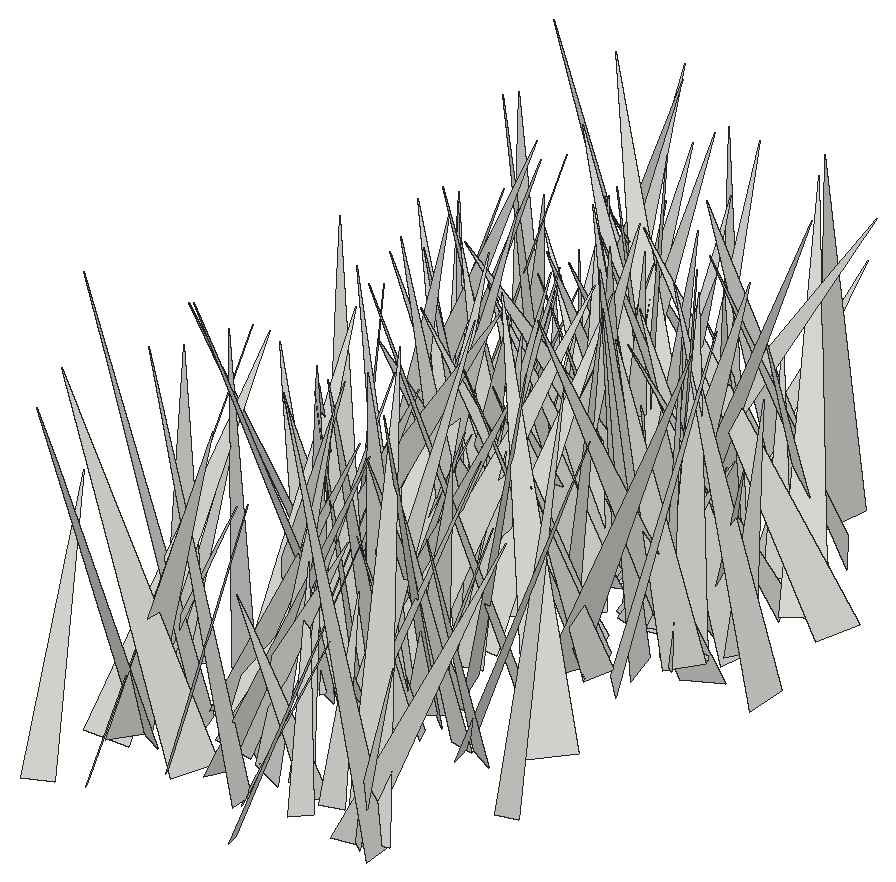
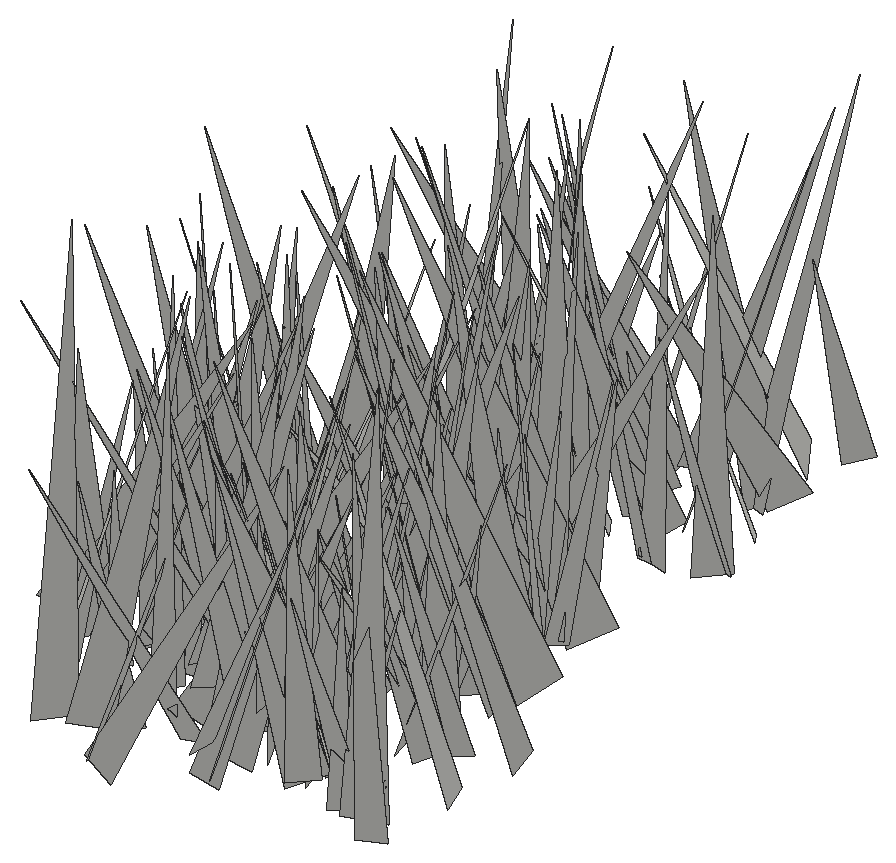
# SketchUp Ruby script. Lengths in inches.
U = 1.inch
M = Sketchup.active_model
def pt(a) = Geom::Point3d.new(a.map { |v| v * U })
def face(e, loops, mat)
  f = e.add_face(loops[0].map { |a| pt(a) })
  loops[1..].each { |l| e.add_face(l.map { |a| pt(a) }).erase! }
  f.material = f.back_material = mat if mat
  f
end
# faces: each face lists its corners as indices into pts; further lists are holes
def faces(e, pts, list, mat = nil) = list.each { |f| face(e, (f[0].is_a?(Array) ? f : [f]).map { |l| l.map { |i| pts[i] } }, mat) }
# xy, xz, yz: faces in a plane at the given z, y or x. An outline is a flat list of corners, or four numbers for a rectangle; further outlines are holes
def ring(l) = l.size == 4 ? [[l[0], l[1]], [l[2], l[1]], [l[2], l[3]], [l[0], l[3]]] : l.each_slice(2).to_a
def flat(e, list, mat, &to3) = list.each { |f| face(e, (f[0].is_a?(Array) ? f : [f]).map { |l| ring(l).map { |u, v| to3.(u, v) } }, mat) }
def xy(e, z, list, mat = nil) = flat(e, list, mat) { |x, y| [x, y, z] }
def xz(e, y, list, mat = nil) = flat(e, list, mat) { |x, z| [x, y, z] }
def yz(e, x, list, mat = nil) = flat(e, list, mat) { |y, z| [x, y, z] }
def lines(e, pts, list) = list.each { |a, b| e.add_line(pt(pts[a]), pt(pts[b])) }
# prism: a flat outline (further loops are holes) pulled along v
def prism(e, loops, v, mat = nil)
  f = face(e, loops, mat); d = Geom::Vector3d.new(v.map { |x| x * U })
  f.pushpull(f.normal.samedirection?(d) ? d.length : -d.length)
end
def box(e, o, s, mat = nil) = prism(e, [[o, [o[0] + s[0], o[1], o[2]], [o[0] + s[0], o[1] + s[1], o[2]], [o[0], o[1] + s[1], o[2]]]], [0, 0, s[2]], mat)
def at(x, y, z, deg = 0) = Geom::Transformation.translation(pt([x, y, z])) * Geom::Transformation.rotation(ORIGIN, Z_AXIS, deg.degrees)
def axes(o, x, y, z) = Geom::Transformation.new([*x, 0, *y, 0, *z, 0, *pt(o).to_a, 1])
def part(name) = M.definitions.add(name)
# library, detail: a bought-in or finely detailed component or shape, given as its bounding box
def library(name, o, s) = part(name).tap { |d| box(d.entities, o, s) }
def detail(e, o, s) = box(e.add_group.entities, o, s)
def put(e, d, t, mat = nil) = e.add_instance(d, t).tap { |i| i.material = mat if mat }
def group(e, t, mat = nil) = e.add_group.tap { |g| g.transformation = t; g.material = mat if mat }.entities
root = M.entities
c1 = part("fur_instance\#9")
p = [[0.8125,0,1.79],[0.67,-0.02,1.48],[0,-0.11,0],[0,0.11,0]]
faces(c1.entities,p,[[0,1,2,3]])
put(root,c1,axes([74.57,65.62,-28.22],[6.72772,1.76518,0.89994],[1.69777,-6.77807,0.60273],[-1.02144,0.36032,6.92927]))
put(root,c1,axes([76.2,71.65,-28.22],[2.05152,-6.96349,2.48946],[-7.36809,-2.14532,0.07104],[-0.63146,2.40909,7.25905]))
put(root,c1,axes([76.23,53.86,-27.1],[4.61817,-3.87726,2.02523],[-4.05143,-4.90172,-0.14567],[-1.64942,1.18414,6.02822]))
put(root,c1,axes([75.16,72.59,-28.22],[0.26156,-6.27199,1.2943],[-6.21893,0.06053,1.55008],[1.52905,1.31908,6.08306]))
put(root,c1,axes([77.24,45.125,-27.1],[-3.56448,3.67904,0.44666],[3.56023,3.5714,-1.00507],[1.02934,0.38746,5.02301]))
put(root,c1,axes([78.23,67.21,-28.22],[-5.39834,-1.72938,0.70035],[-1.70183,5.44274,0.32197],[0.76486,-0.09564,5.65943]))
put(root,c1,axes([79.26,51.24,-27.1],[-7.24522,-3.15461,1.03201],[-3.28219,7.17812,-1.10079],[0.49381,1.42581,7.82516]))
put(root,c1,axes([77.72,70.49,-28.22],[-2.1087,-2.96786,0.97974],[-3.12443,1.97245,-0.74971],[-0.07759,1.23123,3.56269]))
put(root,c1,axes([77.92,64.53,-27.1],[-4.02809,-0.22088,0.67447],[-0.39433,3.92835,-1.06856],[0.59008,1.11738,3.89005]))
put(root,c1,axes([76.2,53.45,-27.1],[1.29664,4.3065,0.97913],[4.41517,-1.23995,-0.39328],[0.1042,-1.05001,4.48024]))
put(root,c1,axes([74.85,68.74,-28.22],[6.72571,2.73267,0.89443],[2.78268,-6.75899,-0.27437],[-0.72399,-0.59256,7.25447]))
put(root,c1,axes([77.43,70.7,-28.22],[-0.62554,4.99616,0.12365],[4.99768,0.62512,0.02455],[-0.009,-0.12574,5.03511]))
put(root,c1,axes([78.375,57.875,-27.1],[-1.43576,4.62376,1.24523],[4.74317,1.1948,1.0324],[-0.65727,-1.47798,4.73019]))
put(root,c1,axes([77.3,60.48,-27.1],[-3.93498,0.71077,2.15609],[1.47172,4.08376,1.33974],[1.72857,-1.85895,3.76754]))
put(root,c1,axes([76.38,62.34,-27.1],[-4.16703,-2.76107,2.92288],[-2.78486,5.0182,0.77013],[2.90022,0.85149,4.93909]))
put(root,c1,axes([77.23,71.6,-28.22],[2.21811,-2.97156,1.30139],[-3.14682,-2.35396,-0.01147],[-0.78819,1.03561,3.7081]))
put(root,c1,axes([77.92,65.62,-28.22],[-2.20554,5.93145,2.00046],[6.2413,2.24627,0.22087],[0.47966,-1.95462,6.32437]))
put(root,c1,axes([75.81,71.11,-27.1],[3.73133,2.74864,1.27928],[3.02044,-3.19509,-1.94493],[0.26177,-2.31318,4.20655]))
put(root,c1,axes([76.375,66.4375,-28.22],[-0.11814,4.24138,1.60816],[4.31681,0.59918,-1.26317],[1.39308,-1.49704,4.05064]))
put(root,c1,axes([77.28,48.58,-27.1],[-4.67484,5.38464,0.57126],[4.73589,4.43174,-3.01759],[2.62527,1.59378,6.46085]))
put(root,c1,axes([76.33,64.45,-27.1],[6.99612,0.8962,1.32294],[0.53893,-6.91662,1.83548],[-1.5043,1.69005,6.81028]))
put(root,c1,axes([78.14,49.53,-27.1],[-2.86218,-6.85746,0.77217],[-6.83354,2.93291,0.71683],[0.96112,0.43167,7.39614]))
put(root,c1,axes([78.7,65.04,-27.1],[2.01081,5.29668,2.07869],[5.40677,-2.46554,1.0522],[-1.77275,-1.51176,5.56697]))
put(root,c1,axes([80.99,57.3,-27.1],[-3.56669,-5.90918,0.59479],[-5.71236,3.22345,-2.22975],[-1.62517,1.63841,6.53207]))
put(root,c1,axes([79.25,68.78,-27.1],[-6.68963,-2.36331,2.10659],[-2.62997,6.88987,-0.62215],[1.76244,1.31094,7.06748]))
put(root,c1,axes([77.18,67.32,-28.22],[3.08965,-1.86478,1.07968],[-2.12915,-2.93231,1.02827],[-0.33144,1.45368,3.45919]))
put(root,c1,axes([75.82,63.17,-27.1],[7.81962,-2.04899,1.63917],[-2.46618,-7.49875,2.3913],[-0.8962,2.75717,7.72182]))
put(root,c1,axes([78.22,54.46,-27.1],[-1.72933,-6.01967,2.37326],[-6.41752,1.90965,0.16749],[0.82719,2.23073,6.26091]))
put(root,c1,axes([77.84,66.42,-27.1],[3.89032,1.8987,0.46131],[1.51623,-3.58179,1.95558],[-1.23244,1.58688,3.86204]))
put(root,c1,axes([80.93,73.32,-27.1],[-7.3033,-3.33888,1.09507],[-3.45877,7.27632,-0.88176],[0.61989,1.26191,7.98178]))
put(root,c1,axes([76.66,51.13,-27.1],[3.8277,2.64651,0.3376],[2.6435,-3.68235,-1.10521],[0.36045,-1.09797,4.52038]))
put(root,c1,axes([78.35,60.38,-27.1],[0.55845,-3.67703,0.59896],[-3.72525,-0.55803,0.04757],[-0.0423,0.59936,3.71889]))
put(root,c1,axes([80.03,63.82,-27.1],[-2.9661,5.6248,1.68099],[5.86235,2.73802,1.18234],[-0.31135,-2.03143,6.24805]))
put(root,c1,axes([78.06,72.44,-27.1],[3.7544,-3.60472,1.46029],[-3.77286,-3.86843,0.15082],[-0.94444,1.12393,5.20257]))
put(root,c1,axes([80.8,48.69,-27.1],[-5.74656,4.30747,2.03787],[4.75581,5.38477,2.02895],[0.29923,-2.86007,6.88916]))
put(root,c1,axes([79.17,70.58,-28.22],[-4.422,-0.95671,1.75223],[-1.16644,4.69405,-0.38074],[1.6202,0.76828,4.50826]))
put(root,c1,axes([77.58,62.09,-27.1],[6.54433,-2.87567,1.841],[-3.10892,-6.66403,0.64215],[-1.41189,1.3447,7.11937]))
put(root,c1,axes([77.62,62.73,-27.1],[3.69637,0.13401,0.11411],[0.12786,-3.69317,0.19555],[-0.12096,0.19138,3.69362]))
put(root,c1,axes([77.38,64.68,-27.1],[2.01974,-4.62687,0.27657],[-4.52399,-1.90214,1.21619],[1.00891,0.73329,4.89981]))
put(root,c1,axes([79.6,67.66,-28.22],[-6.44031,-4.10602,1.97316],[-3.85542,6.73281,1.42663],[2.42663,-0.20036,7.50344]))
put(root,c1,axes([79.36,65.3125,-27.1],[-5.69321,-2.11736,2.09192],[-1.78965,6.04293,1.24584],[2.37833,-0.52131,5.94506]))
put(root,c1,axes([80.4,67.98,-28.22],[-5.18821,0.426,1.12668],[0.56814,5.25845,0.62796],[1.06213,-0.73187,5.16766]))
put(root,c1,axes([77.65,60.375,-27.1],[-1.30326,-6.4856,0.41929],[-6.05179,1.36694,2.33336],[2.36951,-0.07596,6.19006]))
put(root,c1,axes([80.39,58.46,-27.1],[-1.23415,4.06964,0.18802],[4.01431,1.18128,0.78126],[-0.69473,-0.40381,4.18028]))
put(root,c1,axes([79.7,69.08,-28.22],[-7.05102,3.6652,1.50452],[2.87345,6.84526,-3.20935],[2.72774,2.26338,7.26985]))
put(root,c1,axes([78.58,46.01,-27.1],[6.47169,4.71895,0.84374],[4.29058,-6.33416,2.51645],[-2.13805,1.57262,7.60387]))
put(root,c1,axes([77.86,69.9,-27.1],[7.57177,-0.43303,1.80554],[-0.88332,-7.50835,1.90355],[-1.63317,2.05334,7.34137]))
put(root,c1,axes([82.125,57.54,-27.1],[-6.70082,0.16595,0.10129],[0.12128,6.29761,-2.29436],[0.15195,2.29157,6.29797]))
put(root,c1,axes([78.89,59.1,-27.1],[-1.68385,4.77561,0.18208],[4.53538,1.65768,-1.53538],[1.50664,0.34725,4.82539]))
put(root,c1,axes([80.23,59.44,-27.1],[-3.57041,1.71359,0.7726],[1.61509,3.64514,-0.62093],[0.96166,0.24019,3.91135]))
put(root,c1,axes([78.79,69.76,-28.22],[4.20297,-1.11156,0.80651],[-1.18233,-4.24977,0.30429],[-0.69867,0.5049,4.33681]))
put(root,c1,axes([81.92,72.79,-27.1],[-5.15429,0.32159,0.0951],[0.32057,5.15491,-0.05731],[0.09848,0.05128,5.164]))
put(root,c1,axes([77.75,49.14,-27.1],[6.355,-3.28716,0.66061],[-3.33311,-6.3472,0.48096],[-0.36352,0.73183,7.13864]))
put(root,c1,axes([77.41,58.91,-27.1],[3.81653,-4.78014,0.36891],[-4.62204,-3.54318,1.90641],[1.2738,1.46558,5.81217]))
put(root,c1,axes([81.25,55.76,-27.1],[-7.16118,3.19135,1.99245],[3.1192,7.43157,-0.69239],[2.1036,-0.15533,7.80947]))
put(root,c1,axes([81.09,70.15,-27.1],[-3.67286,3.55796,0.5072],[3.52102,3.70767,-0.51167],[0.72023,0.01818,5.08794]))
put(root,c1,axes([80.46,65.18,-27.1],[3.62515,-5.36286,0.15908],[-5.03579,-3.46731,-2.13211],[-1.85105,-1.06996,6.11196]))
put(root,c1,axes([79.2,70.78,-28.22],[5.50822,-3.47682,2.75588],[-4.25576,-5.38219,1.71589],[-1.25366,2.99458,6.28367]))
put(root,c1,axes([82.82,68.71,-28.22],[-3.6214,4.75768,0.36392],[4.63089,3.39426,1.70771],[-1.15013,-1.31374,5.73008]))
put(root,c1,axes([78.59,70.18,-28.22],[4.42426,3.38365,0.88099],[3.49585,-4.30744,-1.01209],[-0.06566,-1.34021,5.47712]))
put(root,c1,axes([80.74,65.16,-28.22],[-4.41847,1.33903,1.10997],[0.76139,4.21375,-2.05244],[1.56375,1.73183,4.13562]))
put(root,c1,axes([78.8125,60.33,-27.1],[3.29309,2.39527,0.08068],[2.3726,-3.23886,-0.68467],[0.3385,-0.60058,4.0141]))
put(root,c1,axes([81.21,64.29,-27.1],[3.41803,-2.18502,2.15563],[-1.95303,-4.03718,-0.99543],[-2.36786,0.1758,3.93273]))
put(root,c1,axes([80.29,52.21,-27.1],[-2.04424,6.85145,0.72305],[6.79433,2.1298,-0.97223],[1.1412,-0.40704,7.08351]))
put(root,c1,axes([83.23,48.0625,-27.1],[-7.26619,-2.16018,0.91047],[-2.32448,7.02333,-1.88745],[0.30351,2.07347,7.34176]))
put(root,c1,axes([81.4,61.94,-27.1],[-6.84332,-0.22544,2.15666],[-0.013,7.14388,0.70553],[2.16837,-0.66867,6.81058]))
put(root,c1,axes([81.04,58.81,-27.1],[-5.5806,3.5391,0.90465],[3.04631,5.42049,-2.4135],[2.01583,1.60617,6.15169]))
put(root,c1,axes([81.13,70.24,-28.22],[2.90611,1.79436,1.69144],[1.585,-3.36196,0.84331],[-1.88904,-0.06039,3.30969]))
put(root,c1,axes([79.44,60.96,-27.1],[7.05742,-1.09775,2.22467],[-1.64487,-7.09246,1.71837],[-1.85705,2.1103,6.93249]))
put(root,c1,axes([79.86,64.58,-28.22],[1.46502,-3.697,0.60293],[-3.73698,-1.39797,0.50827],[0.25762,0.74531,3.94408]))
put(root,c1,axes([78.72,64.59,-27.1],[3.57739,2.98141,0.96801],[3.07785,-3.06266,-1.94177],[0.59384,-2.08684,4.23274]))
put(root,c1,axes([76.67,59.43,-27.1],[6.17977,-5.38552,0.13557],[-5.06059,-5.73249,2.95646],[1.84733,2.31224,7.64543]))
put(root,c1,axes([81.78,71.32,-28.22],[0.31088,-6.10314,0.84199],[-6.04835,-0.46277,-1.12122],[-1.17245,0.76905,6.00731]))
put(root,c1,axes([82.6,63.05,-27.1],[-2.33709,5.71521,1.48586],[5.84354,2.00796,1.46781],[-0.85111,-1.90732,5.99759]))
put(root,c1,axes([81.27,70,-27.1],[-2.39364,-3.13142,1.17859],[-3.27618,2.48779,-0.04385],[0.67935,0.9641,3.94124]))
put(root,c1,axes([81.78,72.84,-28.22],[-0.6438,-6.00502,0.1729],[-5.98541,0.62626,-0.53591],[-0.51472,0.22839,6.0156]))
put(root,c1,axes([83.41,54.36,-27.1],[-4.28269,-7.03673,0.88853],[-7.06243,4.13524,-1.29164],[-0.65353,1.42504,8.13564]))
put(root,c1,axes([78.8125,65.11,-27.1],[1.7793,-6.50243,0.4842],[-6.28195,-1.575,1.93351],[1.74732,0.95904,6.45825]))
put(root,c1,axes([80.44,59.26,-27.1],[3.75823,0.40452,0.85087],[0.18545,-3.74836,0.96295],[-0.9237,0.89332,3.65522]))
put(root,c1,axes([79.92,48.54,-27.1],[4.69401,2.26049,0.88712],[2.32694,-4.7392,-0.23643],[-0.69438,-0.60059,5.20458]))
put(root,c1,axes([79.67,67.94,-28.22],[5.23362,2.8594,0.35445],[2.818,-5.23298,0.60609],[-0.60055,0.36375,5.93293]))
put(root,c1,axes([79.09,52.42,-27.1],[5.6454,-1.61471,0.55375],[-1.70236,-5.46688,1.41409],[-0.12614,1.5134,5.69896]))
put(root,c1,axes([78.53,54.45,-27.1],[5.01746,5.30698,2.27397],[5.71554,-4.13917,-2.95123],[0.81705,-3.63499,6.68051]))
put(root,c1,axes([84,69.34,-27.1],[-6.13421,5.52562,0.24546],[5.52788,6.11218,0.5523],[-0.18784,-0.57446,8.23747]))
put(root,c1,axes([79.4375,71.14,-27.1],[2.86437,6.58912,2.04567],[6.83224,-2.40073,-1.83379],[0.96006,-2.57407,6.94682]))
put(root,c1,axes([82.47,67.83,-28.22],[-0.13118,-4.53208,0.33432],[-4.41868,0.04908,-1.06843],[-1.06148,0.35576,4.40629]))
put(root,c1,axes([80.7,53.5,-27.1],[3.10796,2.24348,0.34109],[2.21254,-3.12436,0.38987],[-0.50422,0.11876,3.81322]))
put(root,c1,axes([82.21,67.47,-27.1],[2.45384,5.3856,0.3895],[5.06414,-2.44383,1.88676],[-1.87372,0.44803,5.60947]))
put(root,c1,axes([83.11,67.75,-27.1],[-5.60277,-1.40853,0.55452],[-1.25772,5.51462,1.29985],[0.84237,-1.13469,5.62898]))
put(root,c1,axes([80.61,55.29,-27.1],[-1.45623,-6.82166,1.9418],[-6.84757,1.86878,1.42991],[1.84835,1.54881,6.82723]))
put(root,c1,axes([84.48,69.91,-28.22],[1.75618,-7.20882,1.45322],[-6.25973,-2.24953,-3.59425],[-3.85938,0.3683,6.49097]))
put(root,c1,axes([82.93,66.03,-28.22],[-5.70691,2.72816,1.15825],[2.57005,5.80682,-1.01437],[1.47624,0.43731,6.24361]))
put(root,c1,axes([82.22,69.49,-27.1],[-4.28945,-4.51982,0.83876],[-4.25056,4.33652,1.63064],[1.75072,-0.54543,6.01408]))
put(root,c1,axes([80.57,62.47,-27.1],[4.17066,5.06918,1.33611],[5.23853,-4.09478,-0.81653],[-0.19883,-1.55319,6.51339]))
put(root,c1,axes([81.83,50.55,-27.1],[4.6203,4.92142,0.32663],[4.69042,-4.52255,1.79463],[-1.52544,1.00021,6.50745]))
put(root,c1,axes([82.35,55.23,-27.1],[4.90048,2.76624,3.25214],[3.64641,-5.28694,-0.99757],[-2.22086,-2.5767,5.5382]))
put(root,c1,axes([84.88,74.38,-28.22],[-1.63485,-6.2778,0.46595],[-5.97391,1.39539,-2.16005],[-1.98499,0.97094,6.117]))
put(root,c1,axes([84.64,64.39,-28.22],[-6.88482,-1.0416,0.48285],[-0.90858,6.73783,1.57954],[0.70182,-1.49517,6.78165]))
put(root,c1,axes([81.07,61.65,-27.1],[3.79421,5.57197,1.64798],[5.81056,-3.63804,-1.07735],[0.00109,-1.96889,6.65448]))
put(root,c1,axes([82.67,55.93,-27.1],[-2.15861,-6.19615,1.53511],[-6.31129,2.3146,0.46773],[0.95736,1.28794,6.5447]))
put(root,c1,axes([82.03,60.75,-27.1],[4.84887,3.21318,0.05137],[2.84684,-4.33809,2.62966],[-1.49084,2.16682,5.18854]))
put(root,c1,axes([85.3125,68.05,-27.1],[-7.32829,2.58062,0.59876],[2.60966,7.33524,0.32553],[0.45582,-0.50666,7.76257]))
put(root,c1,axes([80.65,66.39,-28.22],[1.45839,-7.20301,2.88114],[-7.56056,-0.66269,2.17028],[1.73849,3.16049,7.02141]))
put(root,c1,axes([83.4375,70.14,-27.1],[-3.37227,-0.8607,0.92289],[-0.91034,3.4828,-0.07828],[0.87397,0.30665,3.4795]))
put(root,c1,axes([80.45,58.72,-27.1],[5.56558,-2.4926,0.3103],[-2.49513,-5.39934,1.38077],[0.28926,1.38533,5.93988]))
put(root,c1,axes([82.21,70.1,-27.1],[-0.35457,5.93898,1.63328],[6.05839,0.63143,-0.98081],[1.11129,-1.54746,5.86815]))
put(root,c1,axes([81.29,69.33,-27.1],[1.38948,-7.3294,0.52561],[-7.22169,-1.26322,1.47599],[1.35779,0.7818,7.31247]))
put(root,c1,axes([84.28,68.3,-27.1],[-5.98871,-2.33617,1.80164],[-2.60473,6.10133,-0.74665],[1.38529,1.37273,6.38474]))
put(root,c1,axes([82.04,61.98,-27.1],[4.94298,-3.20176,1.42299],[-3.34359,-5.04595,0.26096],[-1.0472,0.99819,5.88356]))
put(root,c1,axes([80.73,69.58,-28.22],[3.3459,3.39415,0.39754],[3.18536,-2.89609,-2.08314],[1.23764,-1.72213,4.2867]))
put(root,c1,axes([82.32,56.78,-27.1],[3.11086,-6.46121,1.0779],[-6.53922,-3.13316,0.09147],[-0.38422,1.01124,7.17051]))
put(root,c1,axes([82.4375,68.66,-28.22],[5.91489,-2.56905,1.81184],[-2.61095,-6.16477,-0.21752],[-1.75092,0.51416,6.44505]))
put(root,c1,axes([81.48,48.98,-27.1],[6.28882,0.29269,0.74734],[0.08478,-6.11246,1.68051],[-0.79813,1.65699,6.06719]))
put(root,c1,axes([82.47,69.2,-27.1],[5.33637,4.77614,2.80857],[5.34994,-5.45601,-0.88678],[-1.44141,-2.56842,7.10647]))
put(root,c1,axes([84.35,54.84,-27.1],[-0.90978,-4.59674,2.27002],[-5.08569,0.51819,-0.98893],[-0.64715,2.39002,4.58036]))
put(root,c1,axes([82.79,49.875,-27.1],[2.70818,5.99392,1.73773],[6.22026,-2.74585,-0.22279],[-0.5051,-1.67756,6.57356]))
put(root,c1,axes([84.57,52.48,-27.1],[-3.5972,0.42819,0.55364],[0.48536,3.61469,0.35791],[0.50428,-0.42464,3.60487]))
put(root,c1,axes([82.78,60.6,-27.1],[-1.93845,6.02083,0.54238],[5.77969,2.01278,-1.68701],[1.77192,0.02133,6.09606]))
put(root,c1,axes([80.87,50.55,-27.1],[2.62599,-5.06265,0.78885],[-4.77605,-2.09765,2.43674],[1.85526,1.76578,5.15641]))
put(root,c1,axes([85.49,59.4,-27.1],[-6.16047,-5.25921,0.96963],[-5.25018,6.22911,0.42963],[1.01736,0.29959,8.08864]))
put(root,c1,axes([85.1,66.57,-28.22],[0.00148,-6.83986,3.17541],[-7.42007,-0.56775,-1.21947],[-1.34516,3.12424,6.73027]))
put(root,c1,axes([85.04,54.99,-27.1],[-3.24657,-1.58505,0.39086],[-1.61743,3.24104,-0.29141],[0.22149,0.43432,3.60107]))
put(root,c1,axes([83.42,59.38,-27.1],[-1.45732,3.49071,1.72371],[3.67662,1.83923,-0.61623],[1.28012,-1.30851,3.73217]))
put(root,c1,axes([85,49.68,-27.1],[0.84597,-3.78981,1.14812],[-3.67965,-1.18614,-1.20406],[-1.46323,0.79177,3.69169]))
put(root,c1,axes([83.89,50.27,-27.1],[-2.42915,2.39744,1.43013],[2.49267,2.71628,-0.31959],[1.25681,-0.75355,3.39799]))
put(root,c1,axes([84.68,71.32,-27.1],[1.78909,6.44129,2.50482],[6.73985,-2.19865,0.83993],[-1.52927,-2.15428,6.63216]))
put(root,c1,axes([81.8,57.58,-27.1],[-0.75445,7.6495,1.46212],[7.18414,1.25072,-2.83648],[3.00677,-1.06897,7.14412]))
put(root,c1,axes([83.28,53.77,-27.1],[2.96798,6.81466,1.03357],[6.887,-2.97737,-0.1458],[-0.27767,-1.00619,7.4315]))
put(root,c1,axes([82.45,65.79,-28.22],[4.65665,4.64477,2.8893],[5.46904,-4.02795,-2.33914],[-0.10763,-3.71592,6.14709]))
put(root,c1,axes([84.72,57.16,-27.1],[-0.49515,-5.81147,0.35136],[-5.82208,0.49376,-0.03799],[-0.0081,0.35331,5.8324]))
put(root,c1,axes([85.06,67.55,-27.1],[-4.32916,0.66549,1.27706],[0.40908,4.44763,-0.93094],[1.38073,0.76884,4.27993]))
put(root,c1,axes([82.8,58.62,-27.1],[3.70621,1.73352,0.50221],[1.78343,-3.34171,-1.62653],[0.27688,-1.67963,3.75439]))
put(root,c1,axes([85.27,48.52,-27.1],[-3.68366,1.92684,0.76086],[1.83141,3.75443,-0.64122],[0.96827,0.22919,4.10742]))
put(root,c1,axes([83.7,67.48,-27.1],[0.50064,-7.21064,0.91051],[-7.21991,-0.3887,0.89157],[0.83387,0.96363,7.17281]))
put(root,c1,axes([82.26,69.1,-28.22],[5.68552,-4.38043,0.51347],[-4.40819,-5.61738,0.88871],[0.14016,1.01677,7.12204]))
put(root,c1,axes([85.58,73.81,-28.22],[-4.5248,-1.88356,0.71077],[-1.69814,4.51006,1.14127],[1.08134,-0.799,4.76646]))
put(root,c1,axes([86.58,62.52,-27.1],[-4.47388,-2.50611,0.21033],[-2.51468,4.46372,-0.30343],[0.03476,0.36756,5.119]))
put(root,c1,axes([85.8125,66.44,-28.22],[1.42623,8.08681,0.06748],[7.92603,-1.41139,1.61901],[-1.60595,0.21606,8.05043]))
put(root,c1,axes([83.1,48.45,-27.1],[3.88446,1.51086,0.00017],[1.46105,-3.75628,-1.06181],[0.38475,-0.98965,4.03042]))
put(root,c1,axes([86.29,61.76,-27.1],[-4.87517,-3.87645,0.62854],[-3.83008,4.91477,0.6039],[0.86741,-0.08574,6.19915]))
put(root,c1,axes([87.3,68.37,-27.1],[-2.01567,-6.30283,1.43527],[-6.28052,1.55369,-1.99742],[-1.52993,1.92587,6.30864]))
put(root,c1,axes([84.56,45.91,-27.1],[4.68389,2.5085,0.46697],[2.25732,-4.52881,1.68637],[-1.1896,1.28326,5.03861]))
put(root,c1,axes([83.66,70.99,-28.22],[1.01067,5.88602,0.15693],[5.68933,-0.93518,-1.56469],[1.51703,-0.41415,5.76354]))
put(root,c1,axes([85.625,73.92,-27.1],[5.45366,-4.66647,1.60556],[-4.21255,-5.64853,-2.10822],[-2.57063,-0.64365,6.86103]))
put(root,c1,axes([86.49,55.2,-27.1],[-1.41742,-4.71426,1.18858],[-4.85717,1.31918,-0.56008],[-0.21176,1.29675,4.89077]))
put(root,c1,axes([84.28,58.41,-27.1],[6.26752,1.77798,1.53658],[2.00319,-6.33057,-0.84565],[-1.22862,-1.25168,6.45971]))
put(root,c1,axes([84.08,56.71,-27.1],[-3.7888,-7.35051,1.42507],[-6.56657,4.02946,3.32556],[3.59735,-0.38635,7.57137]))
put(root,c1,axes([84.84,66.5,-27.1],[6.67765,-1.57713,2.05629],[-1.75682,-6.93326,0.38749],[-1.90506,0.86558,6.85042]))
put(root,c1,axes([83.48,53.5,-27.1],[5.31801,3.62577,0.57345],[3.65614,-5.14142,-1.39812],[0.32822,-1.47507,6.28273]))
put(root,c1,axes([84.32,56.11,-27.1],[4.15858,-4.6502,0.45845],[-4.67236,-4.14601,0.32855],[-0.05962,0.56087,6.22978]))
put(root,c1,axes([85.68,49.58,-27.1],[-1.6026,3.32948,1.45838],[3.48573,1.8596,-0.41502],[1.03054,-1.11225,3.67172]))
put(root,c1,axes([86.54,64.24,-28.22],[-6.1633,-1.76581,2.36846],[-1.74431,6.59751,0.37966],[2.38433,0.26209,6.40002]))
put(root,c1,axes([82.43,69.09,-27.1],[3.56611,7.00423,0.23479],[6.50816,-3.2121,-3.02618],[2.59966,-1.56674,7.25387]))
put(root,c1,axes([88.74,48.125,-27.1],[-7.60093,-1.69118,1.08047],[-1.85126,7.54274,-1.21718],[0.77483,1.43129,7.69108]))
put(root,c1,axes([84.21,66.53,-28.22],[1.50617,-3.93782,1.16858],[-3.70084,-0.76096,2.20573],[1.78207,1.74788,3.59301]))
put(root,c1,axes([84.49,66.3,-28.22],[1.91277,-3.82749,0.78831],[-3.61325,-1.39793,1.9799],[1.48846,1.5251,3.7932]))
put(root,c1,axes([85.16,70.38,-27.1],[6.59264,-0.88288,1.14982],[-0.53637,-6.4595,-1.88457],[-1.3468,-1.74924,6.37893]))
put(root,c1,axes([88.07,48.43,-27.1],[-0.32528,8.12923,0.88129],[8.06717,0.17507,1.36272],[-1.33486,-0.92294,8.0208]))
put(root,c1,axes([85.71,71.58,-28.22],[1.31447,-3.85278,1.5031],[-4.0825,-0.95693,1.11736],[0.66058,1.75255,3.91449]))
put(root,c1,axes([89.59,69.77,-27.1],[-6.11827,1.22354,0.04324],[1.20265,5.96505,1.37981],[-0.22923,-1.36132,6.08493]))
put(root,c1,axes([87,61.55,-27.1],[3.36953,-3.09183,0.80409],[-2.80421,-3.42236,-1.4084],[-1.53048,-0.53643,4.35081]))
put(root,c1,axes([87.46,70.1,-27.1],[-1.55614,3.71904,0.91385],[3.82438,1.56093,0.15988],[0.20123,-0.90564,4.0283]))
put(root,c1,axes([86.39,67.74,-28.22],[-1.23844,-4.00226,0.78585],[-3.84524,1.41955,1.16979],[1.36007,0.36904,4.02286]))
put(root,c1,axes([89.14,56.52,-27.1],[-5.24663,5.623,0.95369],[5.70188,5.20042,0.70642],[0.12741,-1.17997,7.65808]))
put(root,c1,axes([88.52,66.9,-28.22],[-6.00437,2.1113,1.91932],[2.55574,5.96789,1.43049],[1.26869,-2.0299,6.20191]))
put(root,c1,axes([85.05,66.89,-27.1],[5.41416,-4.66063,0.97473],[-4.76032,-5.26587,1.26282],[0.1044,1.59183,7.03135]))
put(root,c1,axes([87.46,54.98,-27.1],[-1.94034,-4.30134,0.80925],[-4.30819,2.03312,0.47669],[0.77193,0.53502,4.69459]))
put(root,c1,axes([88.58,64.87,-28.22],[0.82289,-7.98079,0.80674],[-7.83354,-0.97405,-1.64552],[-1.72608,0.61581,7.85254]))
put(root,c1,axes([88.16,72.76,-27.1],[-5.39374,-4.42373,0.73063],[-4.15874,5.36317,1.77113],[1.67573,-0.92879,6.74722]))
put(root,c1,axes([85.13,66.97,-27.1],[7.79072,-0.23447,0.87822],[-0.35324,-7.76347,1.06082],[-0.83754,1.09323,7.72172]))
put(root,c1,axes([91.21,68.47,-27.1],[-4.16636,5.9481,1.52453],[5.74666,3.12806,3.50054],[-2.16332,-3.14611,6.36276]))
put(root,c1,axes([88.72,68.73,-27.1],[-5.31145,-3.30369,0.30508],[-3.10318,5.15062,1.7494],[1.17379,-1.33255,6.00546]))
put(root,c1,axes([86.82,65.59,-27.1],[6.37942,2.61315,2.43113],[3.05762,-6.56979,-0.96169],[-1.84118,-1.85616,6.82648]))
put(root,c1,axes([88.2,63.47,-27.1],[2.88835,4.68484,1.93004],[4.79823,-3.24275,0.69058],[-1.62782,-1.24585,5.46016]))
put(root,c1,axes([86.81,74.17,-27.1],[7.55718,-3.05255,1.8054],[-2.7949,-7.74218,-1.39129],[-2.18313,-0.65505,8.03077]))
put(root,c1,axes([88.76,63.72,-27.1],[3.4747,-4.84053,2.29693],[-4.84614,-4.00697,-1.11322],[-2.28507,1.13736,5.85363]))
put(root,c1,axes([89.71,68.57,-27.1],[-3.35316,6.39569,0.22234],[6.39729,3.34326,0.30873],[-0.17041,-0.34016,7.2148]))
put(root,c1,axes([88.4,64.24,-27.1],[-2.28357,5.70644,2.33564],[6.0895,2.47813,-0.10083],[0.96778,-2.12809,6.14557]))
put(root,c1,axes([89.07,70.59,-27.1],[-1.67954,-4.60165,1.09216],[-4.72861,1.65608,-0.29411],[0.09072,1.12742,4.88974]))
put(root,c1,axes([87.66,48.3,-27.1],[2.1321,2.91958,1.28602],[3.18698,-1.87905,-1.01782],[0.14466,-1.63367,3.46899]))
put(root,c1,axes([85.97,60.9,-27.1],[7.43524,-1.67911,0.29476],[-1.69435,-7.42416,0.44731],[-0.18841,0.50147,7.60934]))
put(root,c1,axes([86.73,55.02,-27.1],[6.39935,1.66924,0.57136],[1.67346,-6.42366,0.02366],[-0.55885,-0.12123,6.61343]))
put(root,c1,axes([87.81,61.29,-27.1],[4.5925,4.65986,1.11021],[4.70947,-4.6734,0.13435],[-0.87619,-0.69491,6.5412]))
put(root,c1,axes([87.05,67.5625,-27.1],[4.69242,0.16576,0.10905],[0.19618,-4.2622,-1.96297],[-0.02968,-1.96577,4.26532]))
put(root,c1,axes([88.48,66.9,-28.22],[4.38951,-2.01268,1.547],[-2.15257,-4.58905,0.13732],[-1.34555,0.7756,4.82698]))
put(root,c1,axes([90.93,65.14,-28.22],[-7.32255,-0.11088,1.35528],[-0.08815,7.44603,0.13288],[1.35695,-0.11461,7.32218]))
put(root,c1,axes([87.5,48.12,-27.1],[5.30796,-1.91017,1.71118],[-2.50762,-4.68997,2.54311],[-0.53734,3.01775,5.03546]))
put(root,c1,axes([90.4375,52.57,-27.1],[2.16067,6.65454,0.44246],[6.23565,-2.18071,2.34697],[-2.36543,0.32979,6.59114]))
